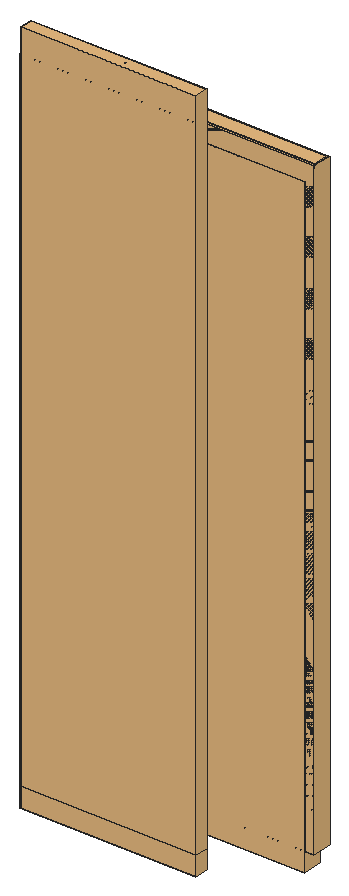
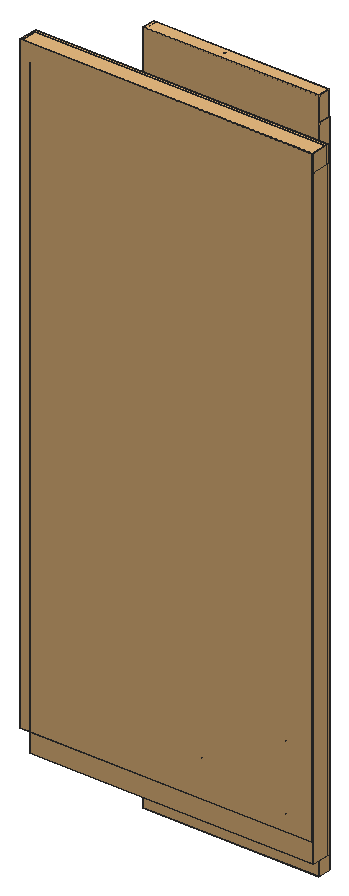
# SketchUp Ruby script. Lengths in inches.
U = 1.inch
M = Sketchup.active_model
def pt(a) = Geom::Point3d.new(a.map { |v| v * U })
def face(e, loops, mat)
  f = e.add_face(loops[0].map { |a| pt(a) })
  loops[1..].each { |l| e.add_face(l.map { |a| pt(a) }).erase! }
  f.material = f.back_material = mat if mat
  f
end
# faces: each face lists its corners as indices into pts; further lists are holes
def faces(e, pts, list, mat = nil) = list.each { |f| face(e, (f[0].is_a?(Array) ? f : [f]).map { |l| l.map { |i| pts[i] } }, mat) }
# xy, xz, yz: faces in a plane at the given z, y or x. An outline is a flat list of corners, or four numbers for a rectangle; further outlines are holes
def ring(l) = l.size == 4 ? [[l[0], l[1]], [l[2], l[1]], [l[2], l[3]], [l[0], l[3]]] : l.each_slice(2).to_a
def flat(e, list, mat, &to3) = list.each { |f| face(e, (f[0].is_a?(Array) ? f : [f]).map { |l| ring(l).map { |u, v| to3.(u, v) } }, mat) }
def xy(e, z, list, mat = nil) = flat(e, list, mat) { |x, y| [x, y, z] }
def xz(e, y, list, mat = nil) = flat(e, list, mat) { |x, z| [x, y, z] }
def yz(e, x, list, mat = nil) = flat(e, list, mat) { |y, z| [x, y, z] }
def lines(e, pts, list) = list.each { |a, b| e.add_line(pt(pts[a]), pt(pts[b])) }
# prism: a flat outline (further loops are holes) pulled along v
def prism(e, loops, v, mat = nil)
  f = face(e, loops, mat); d = Geom::Vector3d.new(v.map { |x| x * U })
  f.pushpull(f.normal.samedirection?(d) ? d.length : -d.length)
end
def box(e, o, s, mat = nil) = prism(e, [[o, [o[0] + s[0], o[1], o[2]], [o[0] + s[0], o[1] + s[1], o[2]], [o[0], o[1] + s[1], o[2]]]], [0, 0, s[2]], mat)
def at(x, y, z, deg = 0) = Geom::Transformation.translation(pt([x, y, z])) * Geom::Transformation.rotation(ORIGIN, Z_AXIS, deg.degrees)
def axes(o, x, y, z) = Geom::Transformation.new([*x, 0, *y, 0, *z, 0, *pt(o).to_a, 1])
def part(name) = M.definitions.add(name)
# library, detail: a bought-in or finely detailed component or shape, given as its bounding box
def library(name, o, s) = part(name).tap { |d| box(d.entities, o, s) }
def detail(e, o, s) = box(e.add_group.entities, o, s)
def put(e, d, t, mat = nil) = e.add_instance(d, t).tap { |i| i.material = mat if mat }
def group(e, t, mat = nil) = e.add_group.tap { |g| g.transformation = t; g.material = mat if mat }.entities
root = M.entities
M.materials.add("green").color = [174, 139, 102]
c1 = part("3DGeom~29_Defintion")
p = [[-0.99,-278.38,-126.59],[-1.52,-278.38,-126.5],[-1.54,-300.55,-125.92],[-1.03,-300.56,-126.01],[-0.92,-237.29,-119.72],[-1.49,-257.76,-123.95],
  [-0.93,-257.75,-124.05],[-1.51,-237.3,-119.62],[-1.01,-325.68,-120.9],[-1.49,-325.66,-120.82],[-1.39,-353.61,-111.43],[-0.95,-353.63,-111.5],
  [-1.3,-191.54,-111.3],[-1.63,-215.67,-114.9],[-1.03,-215.65,-115],[-1.93,-191.55,-111.2],[-3.02,-132.81,-105.31],[-2.625,-163.72,-108.34],
  [-1.96,-163.7,-108.45],[-3.72,-132.84,-105.1875],[-5.18,-69.94,-97.84],[-4.92,-100.91,-101.67],[-4.19,-100.88,-101.79],[-5.9375,-69.97,-97.71],
  [-0.875,-383.21,-98.93],[-1.28,-383.1875,-98.87],[-1.16,-414.39,-83.14],[-0.79,-414.41,-83.19],[-5.45,-19.25,-88.36],[-6.48,-42.06,-93.25],
  [-5.69,-42.04,-93.38],[-6.27,-19.26,-88.22],[-1.87,9.64,-75.67],[-4.96,-2.54,-82.33],[-4.125,-2.57,-82.49],[-2.71,9.7,-75.49],
  [3.6,27.06,-60.84],[0,19.07,-68.14],[0.85,18.99,-68.34],[2.74,27.13,-60.65],[-0.7,-447.22,-64.28],[-1.03,-447.2,-64.23],
  [-0.89,-481.62,-42.16],[-0.6,-481.64,-42.21],[7.12,45.46,-47.33],[5,35.43,-53.44],[5.89,35.39,-53.61],[6.21,45.44,-47.2],
  [5.77,67.15,-39.5],[6.03,56.38,-42.66],[6.95,56.45,-42.77],[4.84,67.03,-39.4],[2.28,88.125,-34.02],[3.13,77.53,-36.72],
  [4.07,77.66,-36.82],[1.33,87.99,-33.92],[0.14,109.59,-25.46],[-0.13,98.6,-30.34],[0.84,98.7,-30.46],[-0.84,109.53,-25.32],
  [1.14,134.61,-9.66],[-0.65,121.53,-18.23],[0.34,121.57,-18.38],[0.13,134.59,-9.49],[3.45,160.94,9.61],[1.25,147.95,0.1],
  [2.27,147.97,-0.07],[2.41,160.92,9.78],[4.85,182.93,26.1875],[3.35,172.78,18.77],[4.4,172.82,18.61],[3.78,182.86,26.33],
  [4,196.81,36.55],[3.57,190.65,32.07],[4.65,190.76,31.96],[2.91,196.65,36.625],[2.24,206.05,44],[2.03,201.51,40.46],
  [3.12,201.7,40.41],[1.14,205.87,44.0625],[1.32,215.82,52.37],[0.46,210.4,47.92],[1.57,210.54,47.82],[0.2,215.73,52.51],
  [2.32,227.77,63.67],[0.49,221.62,57.88],[1.61,221.67,57.7],[1.19,227.73,63.87],[4.19,240.64,76.25],[2.11,234.07,70.16],
  [3.25,234.09,69.95],[3.05,240.61,76.46],[5.3,254.43,87.65],[3.79,247.37,82.45],[4.95,247.41,82.25],[4.13,254.36,87.82],
  [4.65,267.57,96.37],[3.97,260.98,92.36],[5.15,261.09,92.21],[3.47,267.43,96.5],[3.1875,281.38,103.64],[2.75,274.07,100.29],
  [3.95,274.22,100.16],[1.98,281.25,103.78],[2.11,298.65,109.88],[1.3125,289.3125,107.01],[2.53,289.41,106.86],[0.89,298.59,110.05],
  [1.95,318.85,115.22],[0.72,308.52,112.86],[1.96,308.5625,112.68],[0.7,318.83,115.4],[2.17,342.62,119.6],[0.77,330.02,117.71],
  [2.04,330.04,117.52],[0.89,342.6,119.79],[2.37,374.03,123.25],[1,357.1,121.69],[2.29,357.11,121.5],[1.0625,374.02,123.44],
  [2.46,414.46,126.33],[1.08,393.28,125.07],[2.42,393.29,124.875],[1.1,414.46,126.53],[2.55,462.57,128.68],[1.12,437.55,127.8],
  [2.51,437.56,127.59],[1.13,462.5625,128.89],[2.62,518.36,130.3125],[1.14,489.5,129.8],[2.58,489.5,129.59],[1.15,518.36,130.53]]
faces(c1.entities,p,[[0,1,2],[0,2,3],[4,5,6],[4,7,5],[8,9,10],[8,10,11],[12,13,14],[12,15,13],
  [16,17,18],[16,19,17],[20,21,22],[20,23,21],[24,25,26],[24,26,27],[28,29,30],[28,31,29],
  [32,33,34],[32,35,33],[36,37,38],[36,39,37],[40,41,42],[40,42,43],[44,45,46],[44,47,45],
  [48,49,50],[48,51,49],[52,53,54],[52,55,53],[56,57,58],[56,59,57],[60,61,62],[60,63,61],
  [64,65,66],[64,67,65],[68,69,70],[68,71,69],[72,73,74],[72,75,73],[76,77,78],[76,79,77],
  [80,81,82],[80,83,81],[84,85,86],[84,87,85],[88,89,90],[88,91,89],[92,93,94],[92,95,93],
  [96,97,98],[96,99,97],[100,101,102],[100,103,101],[104,105,106],[104,107,105],[108,109,110],[108,111,109],
  [112,113,114],[112,115,113],[116,117,118],[116,119,117],[120,121,122],[120,123,121],[124,125,126],[124,127,125],
  [128,129,130],[128,131,129]],"green")
c2 = part("3DGeom~30_Defintion")
p = [[-0.92,-255.91,-123.16],[-1.51,-276.4,-125.6],[-0.98,-276.4,-125.69],[-1.48,-255.93,-123.07],[-1.03,-298.42,-125.11],[-1.48,-323.34,-119.96],
  [-1.01,-323.36,-120.04],[-1.53,-298.41,-125.02],[-1.02,-214.12,-114.1875],[-1.5,-235.61,-118.77],[-0.92,-235.6,-118.87],[-1.62,-214.14,-114.08],
  [-0.94,-351.11,-110.71],[-1.38,-351.09,-110.63],[-1.27,-380.46,-98.16],[-0.87,-380.48,-98.23],[-1.95,-162.54,-107.68],[-1.92,-190.19,-110.4],
  [-1.29,-190.18,-110.51],[-2.61,-162.56,-107.57],[-4.16,-100.16,-101.07],[-3.69,-131.89,-104.44],[-3,-131.86,-104.56],[-4.88,-100.1875,-100.95],
  [-5.65,-41.74,-92.72],[-5.89,-69.47,-97.02],[-5.14,-69.44,-97.15],[-6.4375,-41.76,-92.58],[-4.1,-2.55,-81.9],[-6.23,-19.12,-87.59],
  [-5.41,-19.11,-87.73],[-4.92,-2.52,-81.75],[-0.79,-411.46,-82.6],[-1.15,-411.43,-82.54],[-1.02,-444.01,-63.78],[-0.7,-444.04,-63.83],
  [0.85,18.85,-67.85],[-2.6875,9.63,-74.96],[-1.85,9.58,-75.14],[0,18.93,-67.66],[5.85,35.14,-53.23],[2.72,26.94,-60.21],
  [3.58,26.86,-60.41],[4.97,35.17,-53.0625],[6.9,56.05,-42.47],[6.17,45.12,-46.86],[7.07,45.14,-46.99],[5.98,55.98,-42.36],
  [-0.6,-478.21,-41.9],[-0.88,-478.19,-41.86],[-0.73,-513.97,-16.8],[-0.49,-513.98,-16.83],[4.04,77.11,-36.55],[4.81,66.56,-39.12],
  [5.73,66.67,-39.22],[3.11,76.97,-36.46],[0.83,98,-30.24],[1.32,87.37,-33.68],[2.26,87.5,-33.78],[-0.13,97.9,-30.13],
  [0.34,120.7,-18.25],[-0.83,108.75,-25.14],[0.14,108.81,-25.28],[-0.65,120.67,-18.1],[2.26,146.92,-0.07],[0.13,133.625,-9.43],
  [1.14,133.65,-9.59],[1.24,146.9,0.1],[4.375,171.59,18.48],[2.39,159.77,9.71],[3.43,159.79,9.54],[3.32,171.55,18.64],
  [4.62,189.41,31.74],[3.75,181.5625,26.14],[4.82,181.63,26],[3.54,189.29,31.85],[3.1,200.26,40.12],[2.89,195.25,36.37],
  [3.97,195.41,36.29],[2.02,200.07,40.17],[1.56,209.04,47.48],[0.46,208.9,47.58],[1.14,204.4,43.75],[2.22,204.59,43.6875],
  [1.6,220.09,57.29],[0.2,214.2,52.14],[1.31,214.28,51.99],[0.49,220.04,57.47],[3.23,232.43,69.45],[1.18,226.11,63.41],
  [2.31,226.15,63.21],[2.1,232.4,69.66],[4.92,245.65,81.67],[3.02,238.9,75.91],[4.17,238.93,75.71],[3.77,245.61,81.86],
  [5.12,259.24,91.55],[4.1,252.55,87.19],[5.27,252.62,87.02],[3.95,259.12,91.7],[3.92,272.26,99.45],[3.44,265.52,95.8125],
  [4.62,265.66,95.68],[2.73,272.12,99.58],[2.51,287.35,106.1],[1.97,279.25,103.04],[3.16,279.38,102.9],[1.3,287.25,106.25],
  [1.95,306.36,111.88],[0.88,296.47,109.26],[2.1,296.52,109.1],[0.72,306.32,112.05],[2.02,327.68,116.68],[0.69,316.56,114.58],
  [1.9375,316.58,114.4],[0.76,327.67,116.87],[2.28,354.5625,120.64],[0.88,340.16,118.94],[2.15,340.18,118.75],[0.99,354.55,120.83],
  [2.4,390.49,123.99],[1.05,371.36,122.5625],[2.35,371.37,122.37],[1.07,390.48,124.18],[2.49,434.4375,126.68],[1.09,411.5,125.625],
  [2.44,411.51,125.43],[1.11,434.43,126.89],[2.57,486.02,128.66],[1.125,459.27,127.97],[2.53,459.27,127.76],[1.14,486.01,128.875]]
faces(c2.entities,p,[[0,1,2],[0,3,1],[4,5,6],[4,7,5],[8,9,10],[8,11,9],[12,13,14],[12,14,15],
  [16,17,18],[16,19,17],[20,21,22],[20,23,21],[24,25,26],[24,27,25],[28,29,30],[28,31,29],
  [32,33,34],[32,34,35],[36,37,38],[36,39,37],[40,41,42],[40,43,41],[44,45,46],[44,47,45],
  [48,49,50],[48,50,51],[52,53,54],[52,55,53],[56,57,58],[56,59,57],[60,61,62],[60,63,61],
  [64,65,66],[64,67,65],[68,69,70],[68,71,69],[72,73,74],[72,75,73],[76,77,78],[76,79,77],
  [80,81,82],[80,82,83],[84,85,86],[84,87,85],[88,89,90],[88,91,89],[92,93,94],[92,95,93],
  [96,97,98],[96,99,97],[100,101,102],[100,103,101],[104,105,106],[104,107,105],[108,109,110],[108,111,109],
  [112,113,114],[112,115,113],[116,117,118],[116,119,117],[120,121,122],[120,123,121],[124,125,126],[124,127,125],
  [128,129,130],[128,131,129]],"green")
c3 = library("3DGeom~31_Defintion",[-9.58,-482.04,-130.39],[19.16,1000,260.06])
c4 = library("3DGeom~32_Defintion",[-7.28,-481.66,-126.81],[15.21,1000,257.33])
c5 = library("3DGeom~33_Defintion",[-9.51,-514.28,-129.47],[19.02,1000,257.51])
c6 = library("3DGeom~34_Defintion",[-7.23,-514,-125.91],[15.11,1000,254.78])
c7 = library("3DGeom~35_Defintion",[-9.58,-482.04,-130.39],[19.16,1000,260.6])
c8 = library("3DGeom~36_Defintion",[-9.51,-514.28,-129.47],[19.02,1000,258.04])
c9 = part("3DGeom~37_Defintion")
p = [[-0.78,-500,-17.86],[-0.32,-499.95,-17.77],[-1.37,-499.29,-16.52],[-1.24,-499.9375,-17.74],[-0.78,-500,-17.86],[-1.37,-499.29,-16.52],
  [-1.24,-499.9375,-17.74],[-1.02,-499.98,-17.83],[-0.78,-500,-17.86],[-0.78,-500,-17.86],[-0.54,-499.99,-17.84],[-0.32,-499.95,-17.77],
  [-0.32,-499.95,-17.77],[0.02,-499.81,-17.51],[-1.37,-499.29,-16.52],[-0.32,-499.95,-17.77],[-0.13,-499.89,-17.66],[0.02,-499.81,-17.51],
  [-1.52,-499.375,-16.67],[-1.42,-499.87,-17.61],[-1.24,-499.9375,-17.74],[-1.52,-499.375,-16.67],[-1.24,-499.9375,-17.74],[-1.37,-499.29,-16.52],
  [-1.64,-499.6875,-17.26],[-1.55,-499.79,-17.45],[-1.42,-499.87,-17.61],[-1.64,-499.6875,-17.26],[-1.42,-499.87,-17.61],[-1.52,-499.375,-16.67],
  [0.02,-499.81,-17.51],[0.16,-499.6,-17.12],[-1.37,-499.29,-16.52],[0.02,-499.81,-17.51],[0.12,-499.71,-17.32],[0.16,-499.6,-17.12],
  [-1.52,-499.375,-16.67],[-1.66,-499.58,-17.06],[-1.64,-499.6875,-17.26],[-1.52,-499.375,-16.67],[-1.62,-499.47,-16.85],[-1.66,-499.58,-17.06],
  [0.16,-499.6,-17.12],[0.06,-499.4,-16.72],[-1.37,-499.29,-16.52],[0.16,-499.6,-17.12],[0.14,-499.5,-16.91],[0.06,-499.4,-16.72],
  [0.06,-499.4,-16.72],[-0.26,-499.25,-16.4375],[-1.37,-499.29,-16.52],[0.06,-499.4,-16.72],[-0.08,-499.3125,-16.5625],[-0.26,-499.25,-16.4375],
  [-0.71,-499.18,-16.3125],[-1.18,-499.23,-16.4],[-1.37,-499.29,-16.52],[-0.26,-499.25,-16.4375],[-0.71,-499.18,-16.3125],[-1.37,-499.29,-16.52],
  [-0.71,-499.18,-16.3125],[-0.96,-499.19,-16.33],[-1.18,-499.23,-16.4],[-0.26,-499.25,-16.4375],[-0.47,-499.2,-16.35],[-0.71,-499.18,-16.3125],
  [0.97,500,115.21],[-2.68,499.88,124.36],[3.67,499.99,115.9],[-1.71,499.99,115.97],[-2.68,499.88,124.36],[0.97,500,115.21],
  [-1.71,499.99,115.97],[0.97,500,115.21],[-0.44,500,115.42],[0.97,500,115.21],[3.67,499.99,115.9],[2.39,500,115.38],
  [3.67,499.99,115.9],[-2.68,499.88,124.36],[5.61,499.97,117.79],[3.67,499.99,115.9],[5.61,499.97,117.79],[4.76,499.98,116.72],
  [-3.53,499.9,123.29],[-2.68,499.88,124.36],[-1.71,499.99,115.97],[-3.53,499.9,123.29],[-1.71,499.99,115.97],[-2.78,499.98,116.82],
  [-4.12,499.95,119.1875],[-3.53,499.9,123.29],[-2.78,499.98,116.82],[-4.12,499.95,119.1875],[-2.78,499.98,116.82],[-3.6,499.97,117.91],
  [5.61,499.97,117.79],[-2.68,499.88,124.36],[6.375,499.93,120.47],[5.61,499.97,117.79],[6.375,499.93,120.47],[6.17,499.95,119.06],
  [-4.29,499.93,120.61],[-3.53,499.9,123.29],[-4.12,499.95,119.1875],[6.375,499.93,120.47],[-2.68,499.88,124.36],[5.68,499.9,123.17],
  [6.375,499.93,120.47],[5.68,499.9,123.17],[6.2,499.91,121.89],[-4.29,499.93,120.61],[-4.08,499.91,122.02],[-3.53,499.9,123.29],
  [5.68,499.9,123.17],[-2.68,499.88,124.36],[3.79,499.87,125.11],[5.68,499.9,123.17],[3.79,499.87,125.11],[4.86,499.88,124.26],
  [1.11,499.86,125.87],[-2.68,499.88,124.36],[-1.59,499.87,125.18],[3.79,499.87,125.11],[-2.68,499.88,124.36],[1.11,499.86,125.87],
  [3.79,499.87,125.11],[1.11,499.86,125.87],[2.53,499.86,125.66],[1.11,499.86,125.87],[-1.59,499.87,125.18],[-0.31,499.86,125.7]]
faces(c9.entities,p,[[0,1,2],[3,4,5],[6,7,8],[9,10,11],[12,13,14],[15,16,17],[18,19,20],[21,22,23],
  [24,25,26],[27,28,29],[30,31,32],[33,34,35],[36,37,38],[39,40,41],[42,43,44],[45,46,47],
  [48,49,50],[51,52,53],[54,55,56],[57,58,59],[60,61,62],[63,64,65],[66,67,68],[69,70,71],
  [72,73,74],[75,76,77],[78,79,80],[81,82,83],[84,85,86],[87,88,89],[90,91,92],[93,94,95],
  [96,97,98],[99,100,101],[102,103,104],[105,106,107],[108,109,110],[111,112,113],[114,115,116],[117,118,119],
  [120,121,122],[123,124,125],[126,127,128],[129,130,131]],"green")
c10 = library("3DGeom~23_Defintion",[-55.93,-500,-156.4375],[111.86,1000,312.875])
c11 = part("3DGeom~24_Defintion")
p = [[-41.625,-500,-145.9375],[-33.19,-499.6,-146.12],[-25.85,-498.52,-142.14],[-53.03,-498.52,-134.4],[-41.625,-500,-145.9375],[-48.66,-495.57,-119.07],
  [-41.625,-500,-145.9375],[-53.03,-498.52,-134.4],[-48.88,-499.6,-141.65],[-48.66,-495.57,-119.07],[-41.625,-500,-145.9375],[-32.89,-494.09,-115.28],
  [-21.48,-495.57,-126.8125],[-41.625,-500,-145.9375],[-25.85,-498.52,-142.14],[-32.89,-494.09,-115.28],[-41.625,-500,-145.9375],[-21.48,-495.57,-126.8125],
  [-21.48,-495.57,-126.8125],[-25.85,-498.52,-142.14],[-21.5625,-497.04,-135.08],[-53.03,-498.52,-134.4],[-48.66,-495.57,-119.07],[-52.95,-497.04,-126.14],
  [-32.89,-494.09,-115.28],[-21.48,-495.57,-126.8125],[-25.625,-494.49,-119.57],[-48.66,-495.57,-119.07],[-32.89,-494.09,-115.28],[-41.32,-494.49,-115.09],
  [36.02,500,126.625],[51.72,497.67,130.14],[44.44,499.375,126.37],[36.02,500,126.625],[36.03,491.3,156.4375],[44.44,490.68,156.18],
  [36.02,500,126.625],[44.44,490.68,156.18],[51.73,491.3,151.97],[36.02,500,126.625],[28.75,493.01,152.67],[36.03,491.3,156.4375],
  [36.02,500,126.625],[51.73,491.3,151.97],[55.93,493.01,144.92],[36.02,500,126.625],[24.54,495.34,145.875],[28.75,493.01,152.67],
  [36.02,500,126.625],[55.93,493.01,144.92],[55.93,495.34,136.93],[36.02,500,126.625],[24.54,497.67,137.89],[24.54,495.34,145.875],
  [36.02,500,126.625],[55.93,495.34,136.93],[51.72,497.67,130.14],[36.02,500,126.625],[28.74,499.375,130.84],[24.54,497.67,137.89]]
faces(c11.entities,p,[[0,1,2],[3,4,5],[6,7,8],[9,10,11],[12,13,14],[15,16,17],[18,19,20],[21,22,23],
  [24,25,26],[27,28,29],[30,31,32],[33,34,35],[36,37,38],[39,40,41],[42,43,44],[45,46,47],
  [48,49,50],[51,52,53],[54,55,56],[57,58,59]],"green")
c12 = part("3DGeom~106_Defintion")
p = [[13,-457.77,-202.36],[12.43,-457.8,-202.3125],[13.01,-486.125,-217.66],[13.55,-486.1,-217.7],[11.89,-399.92,-173.32],[11.84,-429.07,-187.52],
  [12.45,-429.04,-187.5625],[11.24,-399.94,-173.27],[10.74,-340.47,-146.51],[10.02,-340.5,-146.45],[10.64,-370.42,-159.59],[11.32,-370.39,-159.64],
  [9.74,-274.82,-123],[9.45,-308.6875,-134.19],[10.21,-308.66,-134.25],[8.94,-274.85,-122.9375],[8.71,-207.8125,-101.79],[7.83,-207.84,-101.72],
  [8.42,-240.67,-112.26],[9.26,-240.64,-112.32],[7.13,-153.09,-79.54],[7.1,-178.08,-90.92],[8.02,-178.05,-90.99],[6.18,-153.15,-79.48],
  [4,-118.48,-55.33],[4.82,-133.72,-67.51],[5.79,-133.63,-67.55],[3.02,-118.6,-55.3],[0.33,-95.6,-29.9375],[-0.7,-95.73,-29.92],
  [1.08,-106.39,-42.81],[2.09,-106.26,-42.82],[-1.44,-73.6,-2.8],[-2,-85.27,-16.55],[-0.96,-85.15,-16.59],[-2.51,-73.67,-2.71],
  [0.95,-49.78,26.84],[-1.83,-61.59,11.65],[-0.75,-61.55,11.52],[0.95,-49.78,26.84],[-0.16,-49.81,27.01],[5.32,-27.04,58.03],
  [2.02,-38.3,42.73],[3.14,-38.29,42.55],[5.32,-27.04,58.03],[4.18,-27.0625,58.2],[7.55,-5.16,85.82],[5.8,-16.06,72.8],
  [6.97,-16.01,72.65],[6.36,-5.25,85.91],[4.9,15.04,108.74],[3.7,14.85,108.73],[5.55,5,97.6],[6.74,5.15,97.57],
  [0,34.3,128.09],[-1.23,34.1,128.07],[1.28,24.49,118.99],[2.49,24.7,119.02],[-3.26,54.16,141.33],[-4.54,54.09,141.39],
  [-3.34,43.89,135.65],[-2.08,44.05,135.64],[1.2,113.2,138.8],[-0.38,104.875,137.27],[0.95,104.81,137.18],[-0.15,113.16,138.875],
  [0.07,95.73,138.14],[-2.47,86.16,140.63],[-1.16,86.02,140.55],[-1.25,95.85,138.22],[-2.41,75.83,143.01],[-3.7,75.9375,143.09],
  [-4.55,65.2,143.98],[-3.26,65.16,143.89],[-0.4,131.04,151.24],[-0.67,121.83,143.76],[0.69,121.94,143.73],[-1.77,130.9,151.24],
  [-3.3125,149.46,169.92],[-4.71,149.31,169.92],[-3.22,140.1,160.31],[-1.83,140.26,160.32],[-5.28,167.68,186.64],[-5.98,158.46,179.0625],
  [-4.5625,158.59,179.04],[-6.71,167.6,186.71],[-4.84,183.58,197.42],[-6.74,175.84,192.46],[-5.3,175.86,192.35],[-6.28,183.61,197.56],
  [-3.32,198.87,205.72],[-5.56,191.21,202.02],[-4.1,191.16,201.87],[-4.79,198.92,205.87],[-2.54,215.74,211.62],[-4.2,207,209.1],
  [-2.73,206.98,208.96],[-4.03,215.71,211.74],[-3.51,234.5625,213.875],[-4.36,225.09,213.4375],[-2.87,225.16,213.32],[-5.02,234.48,213.99],
  [-5.16,253.86,213.61],[-6.6875,253.77,213.74],[-5.84,243.98,213.93],[-4.32,244.07,213.8125],[-6.4,274.98,214.6],[-7.43,264.02,213.86],
  [-5.89,264.1,213.73],[-7.96,274.93,214.73],[-6.84,297.22,218.75],[-8.26,286.04,216.51],[-6.68,286.08,216.38],[-8.43,297.18,218.89],
  [-6.9375,322.55,224.28],[-8.52,309.11,221.61],[-6.91,309.14,221.48],[-8.56,322.52,224.42],[-6.99,356.56,229.06],[-8.59,338.11,227.04],
  [-6.95,338.125,226.9],[-8.65,356.54,229.2],[-7.09,400.64,232.43],[-8.73,377.54,230.99],[-7.05,377.56,230.84],[-8.81,400.63,232.57],
  [-7.16,453.07,235],[-8.875,425.8,233.96],[-7.13,425.81,233.8125],[-8.93,453.07,235.16],[-7.18,513.875,236.79],[-8.98,482.42,236.15],
  [-7.17,482.43,236],[-9.02,513.875,236.95]]
faces(c12.entities,p,[[0,1,2],[0,2,3],[4,5,6],[4,7,5],[8,9,10],[8,10,11],[12,13,14],[12,15,13],
  [16,17,18],[16,18,19],[20,21,22],[20,23,21],[24,25,26],[24,27,25],[28,29,30],[28,30,31],
  [32,33,34],[32,35,33],[36,37,38],[39,40,37],[41,42,43],[44,45,42],[46,47,48],[46,49,47],
  [50,51,52],[50,52,53],[54,55,56],[54,56,57],[58,59,60],[58,60,61],[62,63,64],[62,65,63],
  [66,67,68],[66,69,67],[70,71,72],[70,72,73],[74,75,76],[74,77,75],[78,79,80],[78,80,81],
  [82,83,84],[82,85,83],[86,87,88],[86,89,87],[90,91,92],[90,93,91],[94,95,96],[94,97,95],
  [98,99,100],[98,101,99],[102,103,104],[102,104,105],[106,107,108],[106,109,107],[110,111,112],[110,113,111],
  [114,115,116],[114,117,115],[118,119,120],[118,121,119],[122,123,124],[122,125,123],[126,127,128],[126,129,127],
  [130,131,132],[130,133,131]],"green")
c13 = part("3DGeom~107_Defintion")
p = [[13.6,-487.82,-218.47],[13.05,-487.84,-218.43],[13.63,-515.87,-234.39],[14.13,-515.85,-234.43],[12.5,-430.56,-188.23],[12.47,-459.41,-203.03],
  [13.05,-459.39,-203.07],[11.88,-430.58,-188.18],[11.36,-371.7,-160.2],[10.67,-371.73,-160.15],[11.28,-401.36,-173.89],[11.93,-401.33,-173.94],
  [10.25,-309.75,-134.72],[9.49,-309.78,-134.66],[10.06,-341.7,-146.97],[10.78,-341.67,-147.02],[9.29,-241.49,-112.72],[8.45,-241.52,-112.65],
  [8.97,-275.82,-123.37],[9.77,-275.8,-123.4375],[8.05,-178.67,-91.3125],[7.86,-208.57,-102.08],[8.74,-208.55,-102.15],[7.13,-178.71,-91.24],
  [5.81,-134.1,-67.79],[4.83,-134.1875,-67.74],[6.2,-153.69,-79.76],[7.16,-153.63,-79.82],[2.09,-106.64,-42.97],[1.09,-106.77,-42.96],
  [3.03,-119.01,-55.5],[4.02,-118.9,-55.53],[-0.96,-85.46,-16.65],[-2.01,-85.57,-16.6],[-0.7,-96.07,-30.02],[0.33,-95.9375,-30.04],
  [-0.75,-61.77,11.56],[-2.52,-73.93,-2.72],[-1.45,-73.86,-2.81],[-1.84,-61.81,11.7],[3.15,-38.42,42.7],[-0.16,-49.98,27.1],
  [0.95,-49.96,26.9375],[2.03,-38.4375,42.88],[6.99,-16.07,72.91],[4.19,-27.16,58.41],[5.34,-27.14,58.23],[5.82,-16.12,73.06],
  [6.77,5.17,97.91],[6.39,-5.26,86.21],[7.58,-5.17,86.12],[5.56,5.02,97.95],[2.5,24.78,119.4375],[1.28,24.58,119.41],
  [3.71,14.9,109.11],[4.92,15.09,109.12],[-2.09,44.21,136.12],[-3.35,44.05,136.13],[-1.23,34.22,128.52],[0,34.42,128.54],
  [0.96,105.18,137.67],[-1.25,96.19,138.71],[0.07,96.06,138.625],[-0.38,105.24,137.76],[0.7,122.37,144.24],[-0.15,113.56,139.37],
  [1.21,113.6,139.29],[-0.67,122.26,144.27],[-1.17,86.33,141.05],[-3.72,76.2,143.59],[-2.41,76.09,143.51],[-2.48,86.46,141.125],
  [-3.27,65.39,144.4],[-4.56,54.28,141.89],[-3.27,54.35,141.83],[-4.57,65.43,144.49],[-1.84,140.75,160.88],[-3.23,140.59,160.875],
  [-1.78,131.36,151.78],[-0.41,131.5,151.77],[-4.58,159.15,179.67],[-6,159.02,179.69],[-4.73,149.83,170.52],[-3.33,149.99,170.52],
  [-5.32,176.48,193.03],[-6.74,168.19,187.37],[-5.3,168.27,187.3],[-6.76,176.46,193.14],[-4.12,191.83,202.58],[-6.31,184.26,198.26],
  [-4.85,184.23,198.12],[-5.58,191.88,202.74],[-2.73,207.71,209.7],[-4.8,199.62,206.59],[-3.33,199.57,206.44],[-4.22,207.73,209.84],
  [-2.875,225.96,214.07],[-4.05,216.47,212.49],[-2.55,216.5,212.36],[-4.38,225.89,214.19],[-5.91,265.03,214.49],[-6.71,254.67,214.49],
  [-5.17,254.76,214.37],[-7.46,264.96,214.61],[-4.33,244.9375,214.57],[-5.86,244.84,214.6875],[-5.03,235.3,214.75],[-3.52,235.39,214.63],
  [-6.71,287.09,217.15],[-7.99,275.9,215.49],[-6.42,275.95,215.36],[-8.29,287.05,217.28],[-6.9375,310.23,222.26],[-8.46,298.23,219.66],
  [-6.87,298.27,219.53],[-8.55,310.2,222.39],[-6.97,339.32,227.7],[-8.59,323.66,225.21],[-6.96,323.68,225.07],[-8.62,339.3,227.84],
  [-7.07,378.89,231.66],[-8.68,357.8,230.01],[-7.02,357.82,229.87],[-8.76,378.88,231.8],[-7.16,427.3125,234.64],[-8.84,402.04,233.39],
  [-7.12,402.05,233.25],[-8.91,427.31,234.79],[-7.2,484.13,236.83],[-8.96,454.67,235.99],[-7.18,454.67,235.83],[-9.01,484.125,236.99]]
faces(c13.entities,p,[[0,1,2],[0,2,3],[4,5,6],[4,7,5],[8,9,10],[8,10,11],[12,13,14],[12,14,15],
  [16,17,18],[16,18,19],[20,21,22],[20,23,21],[24,25,26],[24,26,27],[28,29,30],[28,30,31],
  [32,33,34],[32,34,35],[36,37,38],[36,39,37],[40,41,42],[40,43,41],[44,45,46],[44,47,45],
  [48,49,50],[48,51,49],[52,53,54],[52,54,55],[56,57,58],[56,58,59],[60,61,62],[60,63,61],
  [64,65,66],[64,67,65],[68,69,70],[68,71,69],[72,73,74],[72,75,73],[76,77,78],[76,78,79],
  [80,81,82],[80,82,83],[84,85,86],[84,87,85],[88,89,90],[88,91,89],[92,93,94],[92,95,93],
  [96,97,98],[96,99,97],[100,101,102],[100,103,101],[104,105,106],[104,106,107],[108,109,110],[108,111,109],
  [112,113,114],[112,115,113],[116,117,118],[116,119,117],[120,121,122],[120,123,121],[124,125,126],[124,127,125],
  [128,129,130],[128,131,129]],"green")
c14 = library("3DGeom~108_Defintion",[-15.55,-485.98,-221.31],[30.67,1000,457.14])
c15 = library("3DGeom~109_Defintion",[-10.83,-486.12,-217.86],[24.87,1000,454.81])
c16 = library("3DGeom~110_Defintion",[-15.46,-515.69,-237.75],[31.06,1000,473.61])
c17 = library("3DGeom~111_Defintion",[-10.8,-515.86,-234.58],[25.39,1000,471.56])
c18 = library("3DGeom~112_Defintion",[-15.55,-486.02,-221.29],[30.67,1000,457.87])
c19 = library("3DGeom~113_Defintion",[-15.46,-515.73,-237.74],[31.06,1000,474.35])
c20 = part("3DGeom~114_Defintion")
p = [[13.375,-498.625,-230.47],[14.29,-498.73,-230.21],[11.9375,-499.79,-227.73],[12.4375,-498.72,-230.29],[13.375,-498.625,-230.47],[11.9375,-499.79,-227.73],
  [12.4375,-498.72,-230.29],[12.89,-498.65,-230.4375],[13.375,-498.625,-230.47],[13.375,-498.625,-230.47],[13.86,-498.65,-230.39],[14.29,-498.73,-230.21],
  [11.67,-499.65,-228.07],[12.4375,-498.72,-230.29],[11.9375,-499.79,-227.73],[11.67,-499.65,-228.07],[12.06,-498.82,-230.05],[12.4375,-498.72,-230.29],
  [14.29,-498.73,-230.21],[14.92,-498.98,-229.58],[11.9375,-499.79,-227.73],[14.29,-498.73,-230.21],[14.65,-498.83,-229.93],[14.92,-498.98,-229.58],
  [11.5,-499.49,-228.48],[12.06,-498.82,-230.05],[11.67,-499.65,-228.07],[11.5,-499.49,-228.48],[11.75,-498.96,-229.73],[12.06,-498.82,-230.05],
  [11.75,-498.96,-229.73],[11.5,-499.49,-228.48],[11.46,-499.3,-228.92],[11.75,-498.96,-229.73],[11.46,-499.3,-228.92],[11.55,-499.12,-229.35],
  [14.92,-498.98,-229.58],[15.125,-499.32,-228.74],[11.9375,-499.79,-227.73],[14.92,-498.98,-229.58],[15.08,-499.14,-229.18],[15.125,-499.32,-228.74],
  [15.125,-499.32,-228.74],[14.83,-499.67,-227.92],[11.9375,-499.79,-227.73],[15.125,-499.32,-228.74],[15.04,-499.51,-228.31],[14.83,-499.67,-227.92],
  [14.83,-499.67,-227.92],[14.15,-499.91,-227.36],[11.9375,-499.79,-227.73],[14.83,-499.67,-227.92],[14.53,-499.81,-227.6],[14.15,-499.91,-227.36],
  [13.21,-500,-227.18],[12.3,-499.9,-227.45],[11.9375,-499.79,-227.73],[14.15,-499.91,-227.36],[13.21,-500,-227.18],[11.9375,-499.79,-227.73],
  [13.21,-500,-227.18],[12.73,-499.97,-227.27],[12.3,-499.9,-227.45],[14.15,-499.91,-227.36],[13.7,-499.98,-227.22],[13.21,-500,-227.18],
  [-8.13,500,217.125],[-13.4,499.85,228.29],[-4.81,499.99,218.2],[-11.54,499.99,217.875],[-13.4,499.85,228.29],[-8.13,500,217.125],
  [-11.54,499.99,217.875],[-8.13,500,217.125],[-9.91,500,217.28],[-8.13,500,217.125],[-4.81,499.99,218.2],[-6.37,500,217.45],
  [-14.375,499.87,226.89],[-13.4,499.85,228.29],[-11.54,499.99,217.875],[-14.375,499.87,226.89],[-11.54,499.99,217.875],[-12.94,499.97,218.85],
  [-4.81,499.99,218.2],[-13.4,499.85,228.29],[-2.53,499.96,220.71],[-4.81,499.99,218.2],[-2.53,499.96,220.71],[-3.5,499.97,219.31],
  [-14.97,499.89,225.26],[-14.375,499.87,226.89],[-12.94,499.97,218.85],[-14.97,499.89,225.26],[-12.94,499.97,218.85],[-14.05,499.96,220.15],
  [-15.125,499.91,223.48],[-14.97,499.89,225.26],[-14.05,499.96,220.15],[-15.125,499.91,223.48],[-14.05,499.96,220.15],[-14.8,499.9375,221.72],
  [-2.53,499.96,220.71],[-13.4,499.85,228.29],[-1.77,499.91,224.12],[-2.53,499.96,220.71],[-1.77,499.91,224.12],[-1.93,499.9375,222.34],
  [-1.77,499.91,224.12],[-13.4,499.85,228.29],[-2.85,499.87,227.44],[-1.77,499.91,224.12],[-2.85,499.87,227.44],[-2.1,499.89,225.88],
  [-2.85,499.87,227.44],[-13.4,499.85,228.29],[-5.36,499.84,229.72],[-2.85,499.87,227.44],[-5.36,499.84,229.72],[-3.96,499.85,228.74],
  [-8.77,499.83,230.47],[-13.4,499.85,228.29],[-12.09,499.84,229.4],[-5.36,499.84,229.72],[-13.4,499.85,228.29],[-8.77,499.83,230.47],
  [-8.77,499.83,230.47],[-12.09,499.84,229.4],[-10.53,499.83,230.15],[-5.36,499.84,229.72],[-8.77,499.83,230.47],[-6.99,499.83,230.32]]
faces(c20.entities,p,[[0,1,2],[3,4,5],[6,7,8],[9,10,11],[12,13,14],[15,16,17],[18,19,20],[21,22,23],
  [24,25,26],[27,28,29],[30,31,32],[33,34,35],[36,37,38],[39,40,41],[42,43,44],[45,46,47],
  [48,49,50],[51,52,53],[54,55,56],[57,58,59],[60,61,62],[63,64,65],[66,67,68],[69,70,71],
  [72,73,74],[75,76,77],[78,79,80],[81,82,83],[84,85,86],[87,88,89],[90,91,92],[93,94,95],
  [96,97,98],[99,100,101],[102,103,104],[105,106,107],[108,109,110],[111,112,113],[114,115,116],[117,118,119],
  [120,121,122],[123,124,125],[126,127,128],[129,130,131]],"green")
g1 = group(root,at(15.3125,38.42,26.21))
put(g1,c1,axes([1.84,0.12,11.26],[0,0.0132,0],[0,0,-0.0132],[-0.0132,0,0]),"green")
put(g1,c2,axes([1.84,0.12,11.26],[0,0.01329,0],[0,0,-0.01329],[-0.01329,0,0]),"green")
put(g1,c3,axes([1.84,0.12,11.26],[0,0.01321,0],[0,0,-0.01321],[-0.01321,0,0]),"green")
put(g1,c4,axes([1.84,0.12,11.26],[0,0.0132,0],[0,0,-0.0132],[-0.0132,0,0]),"green")
put(g1,c5,axes([1.84,0.12,11.26],[0,0.01331,0],[0,0,-0.01331],[-0.01331,0,0]),"green")
put(g1,c6,axes([1.84,0.12,11.26],[0,0.01329,0],[0,0,-0.01329],[-0.01329,0,0]),"green")
put(g1,c7,axes([1.84,0.12,11.26],[0,0.01321,0],[0,0,-0.01321],[-0.01321,0,0]),"green")
put(g1,c8,axes([1.84,0.12,11.26],[0,0.01331,0],[0,0,-0.01331],[-0.01331,0,0]),"green")
put(g1,c9,axes([1.84,0.12,11.26],[0,0.01369,0],[0,0,-0.01369],[-0.01369,0,0]),"green")
g2 = group(root,at(15.3125,38.42,26.21))
put(g2,c10,axes([1.92,0.11,9.55],[0,0.00091,0],[0,0,-0.00091],[-0.00091,0,0]),"green")
put(g2,c11,axes([1.92,0.11,9.55],[0,0.00091,0],[0,0,-0.00091],[-0.00091,0,0]),"green")
g3 = group(root,at(15.3125,38.42,26.21))
put(g3,c12,axes([2.7,0.5625,11.18],[0,0.01211,0],[0,0,-0.01211],[-0.01211,0,0]),"green")
put(g3,c13,axes([2.7,0.5625,11.18],[0,0.01207,0],[0,0,-0.01207],[-0.01207,0,0]),"green")
put(g3,c14,axes([2.7,0.5625,11.18],[0,0.01211,0],[0,0,-0.01211],[-0.01211,0,0]),"green")
put(g3,c15,axes([2.7,0.5625,11.18],[0,0.01211,0],[0,0,-0.01211],[-0.01211,0,0]),"green")
put(g3,c16,axes([2.7,0.5625,11.18],[0,0.01207,0],[0,0,-0.01207],[-0.01207,0,0]),"green")
put(g3,c17,axes([2.7,0.5625,11.18],[0,0.01207,0],[0,0,-0.01207],[-0.01207,0,0]),"green")
put(g3,c18,axes([2.7,0.5625,11.18],[0,0.01211,0],[0,0,-0.01211],[-0.01211,0,0]),"green")
put(g3,c19,axes([2.7,0.5625,11.18],[0,0.01207,0],[0,0,-0.01207],[-0.01207,0,0]),"green")
put(g3,c20,axes([2.7,0.5625,11.18],[0,0.01245,0],[0,0,-0.01245],[-0.01245,0,0]),"green")
